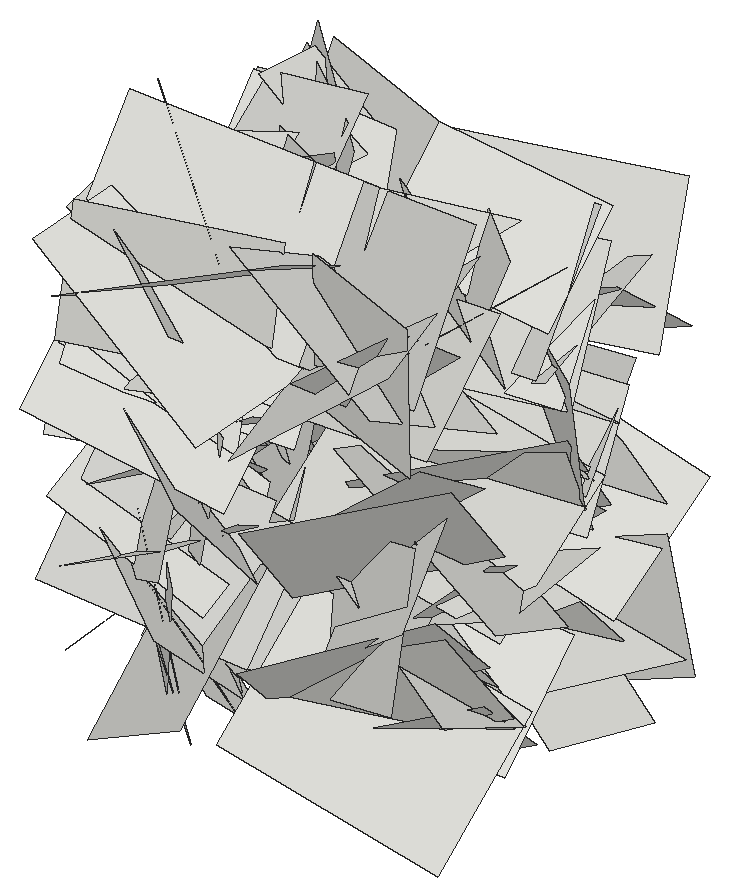
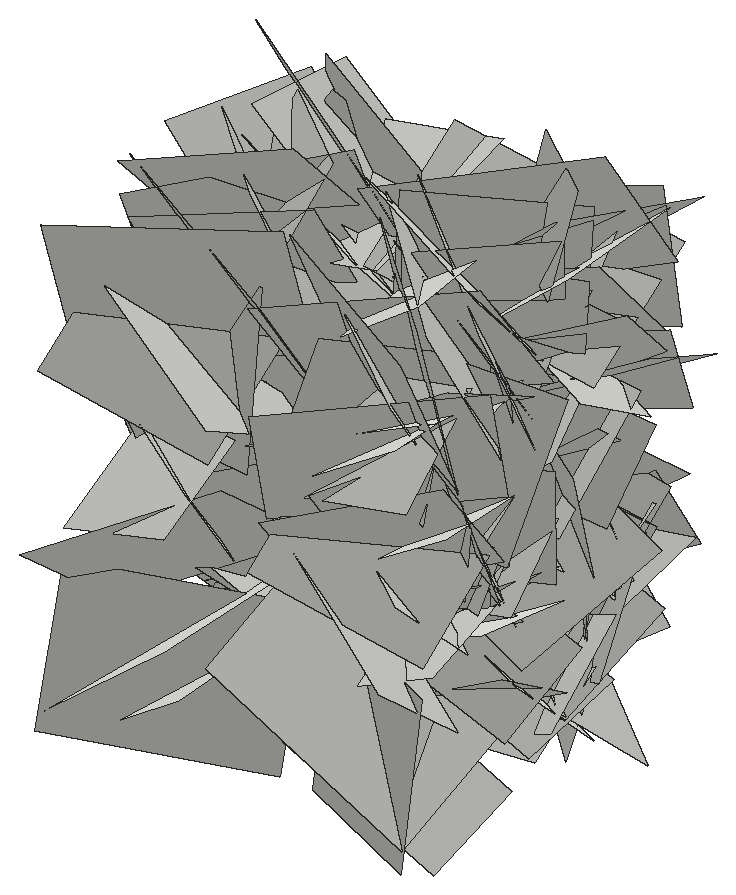
# SketchUp Ruby script. Lengths in inches.
U = 1.inch
M = Sketchup.active_model
def pt(a) = Geom::Point3d.new(a.map { |v| v * U })
def face(e, loops, mat)
  f = e.add_face(loops[0].map { |a| pt(a) })
  loops[1..].each { |l| e.add_face(l.map { |a| pt(a) }).erase! }
  f.material = f.back_material = mat if mat
  f
end
# faces: each face lists its corners as indices into pts; further lists are holes
def faces(e, pts, list, mat = nil) = list.each { |f| face(e, (f[0].is_a?(Array) ? f : [f]).map { |l| l.map { |i| pts[i] } }, mat) }
# xy, xz, yz: faces in a plane at the given z, y or x. An outline is a flat list of corners, or four numbers for a rectangle; further outlines are holes
def ring(l) = l.size == 4 ? [[l[0], l[1]], [l[2], l[1]], [l[2], l[3]], [l[0], l[3]]] : l.each_slice(2).to_a
def flat(e, list, mat, &to3) = list.each { |f| face(e, (f[0].is_a?(Array) ? f : [f]).map { |l| ring(l).map { |u, v| to3.(u, v) } }, mat) }
def xy(e, z, list, mat = nil) = flat(e, list, mat) { |x, y| [x, y, z] }
def xz(e, y, list, mat = nil) = flat(e, list, mat) { |x, z| [x, y, z] }
def yz(e, x, list, mat = nil) = flat(e, list, mat) { |y, z| [x, y, z] }
def lines(e, pts, list) = list.each { |a, b| e.add_line(pt(pts[a]), pt(pts[b])) }
# prism: a flat outline (further loops are holes) pulled along v
def prism(e, loops, v, mat = nil)
  f = face(e, loops, mat); d = Geom::Vector3d.new(v.map { |x| x * U })
  f.pushpull(f.normal.samedirection?(d) ? d.length : -d.length)
end
def box(e, o, s, mat = nil) = prism(e, [[o, [o[0] + s[0], o[1], o[2]], [o[0] + s[0], o[1] + s[1], o[2]], [o[0], o[1] + s[1], o[2]]]], [0, 0, s[2]], mat)
def at(x, y, z, deg = 0) = Geom::Transformation.translation(pt([x, y, z])) * Geom::Transformation.rotation(ORIGIN, Z_AXIS, deg.degrees)
def axes(o, x, y, z) = Geom::Transformation.new([*x, 0, *y, 0, *z, 0, *pt(o).to_a, 1])
def part(name) = M.definitions.add(name)
# library, detail: a bought-in or finely detailed component or shape, given as its bounding box
def library(name, o, s) = part(name).tap { |d| box(d.entities, o, s) }
def detail(e, o, s) = box(e.add_group.entities, o, s)
def put(e, d, t, mat = nil) = e.add_instance(d, t).tap { |i| i.material = mat if mat }
def group(e, t, mat = nil) = e.add_group.tap { |g| g.transformation = t; g.material = mat if mat }.entities
root = M.entities
c1 = part("Component\#6")
p = [[0.01,0,0],[0,3.24,4.54],[4.32,3.24,4.54],[4.33,0,0]]
faces(c1.entities,p,[[0,1,2,3]])
put(root,c1,axes([410.71,164.95,29.96],[-0.04265,0.57286,-0.52342],[0.15347,-0.50938,-0.56862],[0.80809,0.12697,0.08036]))
put(root,c1,axes([410.71,167.51,23.32],[-0.04127,-0.8056,0.43064],[-0.05085,0.43224,0.80425],[0.96695,-0.01165,0.06068]))
put(root,c1,axes([410.71,163.99,40.83],[0.08038,0.23372,-0.81219],[-0.10222,-0.80774,-0.24144],[0.89001,-0.11388,0.04562]))
put(root,c1,axes([410.71,164.8,26.41],[0.06555,-0.88967,-0.10275],[-0.1194,-0.1099,0.88381],[0.94178,0.04799,0.1192]))
put(root,c1,axes([414.68,169.82,24.93],[-0.00586,-0.68753,0.27068],[-0.05817,0.27032,0.6855],[-0.78107,-0.01497,-0.05308]))
put(root,c1,axes([414.68,164.96,33.58],[-0.03363,-0.67551,-0.53197],[0.14584,-0.52946,0.66412],[-0.89967,-0.06058,0.12754]))
put(root,c1,axes([410.71,168.875,35.8],[0.07444,0.7996,-0.0855],[0.00091,-0.0859,-0.80263],[0.85241,-0.06974,0.00832]))
put(root,c1,axes([410.71,164.5,23.79],[0.04443,0.667,0.37408],[0.11412,0.36576,-0.66423],[0.80255,-0.08894,0.07374]))
put(root,c1,axes([410.71,162.92,24.26],[0.16568,0.16434,-0.80239],[-0.1251,-0.80382,-0.18763],[0.85913,-0.14874,0.12742]))
put(root,c1,axes([410.71,162.61,28.57],[-0.04222,-0.49534,0.62953],[0.20196,0.60636,0.48917],[0.82474,-0.17384,-0.08755]))
put(root,c1,axes([410.71,162.43,26.35],[0.02315,-0.70596,0.51236],[-0.01203,0.51225,0.70629],[0.92456,0.02434,-0.00364]))
put(root,c1,axes([414.68,171.89,34.33],[0.10287,-0.74562,-0.1631],[-0.15609,-0.17961,0.73351],[-0.79385,-0.06131,-0.16536]))
put(root,c1,axes([410.71,171.21,38.93],[-0.24063,-0.51313,-1.11059],[-0.16085,-1.10901,0.54342],[1.28679,-0.23458,-0.13976]))
put(root,c1,axes([410.71,166.53,31.68],[-0.02185,0.89564,-0.0065],[0.05171,-0.00537,-0.89456],[0.948,0.02094,0.04865]))
put(root,c1,axes([410.71,158.45,30.92],[-0.16236,0.46297,0.88251],[0.09478,0.89566,-0.45434],[1.05211,-0.00924,0.17712]))
put(root,c1,axes([410.71,163.85,33.45],[-0.03445,-0.73428,-0.4148],[0.17499,-0.41262,0.71747],[0.87664,0.05351,-0.15952]))
put(root,c1,axes([414.68,168.18,25.35],[-0.0356,-0.79141,-0.13903],[0.13499,-0.14264,0.78117],[-0.84098,0.01061,0.13127]))
put(root,c1,axes([414.68,167.69,34.89],[-0.01272,-0.59445,-0.3878],[-0.01652,-0.38754,0.59453],[-0.75216,0.01856,-0.0065]))
put(root,c1,axes([410.71,171.77,39.47],[-0.25632,-0.1505,-1.28885],[-0.2021,-1.29268,0.18672],[1.36053,-0.22038,-0.21508]))
put(root,c1,axes([410.71,166.33,22.3],[-0.05809,-0.87115,0.26873],[0.09257,0.26296,0.87026],[0.96191,-0.07791,-0.06752]))
put(root,c1,axes([410.71,162.32,28.44],[0.12821,-0.42216,-0.69512],[-0.01339,-0.70366,0.42514],[0.86197,0.05186,0.11]))
put(root,c1,axes([414.68,169.92,30.86],[-0.08798,0.07784,-0.70174],[0.08853,-0.70052,-0.08758],[-0.74315,-0.09267,0.07264]))
put(root,c1,axes([410.71,164.2,31.01],[-0.06613,-0.18181,-0.96198],[0.02897,-0.96387,0.1804],[1.03734,0.01533,-0.06637]))
put(root,c1,axes([410.71,161.79,25.53],[0.01152,-0.82607,0.19056],[0.15176,0.18963,0.81386],[0.88572,-0.02175,-0.14193]))
put(root,c1,axes([414.68,169.17,27.35],[-0.00515,-0.4485,-0.48712],[-0.04455,-0.48594,0.44784],[-0.70046,0.0342,-0.02491]))
put(root,c1,axes([414.68,158.39,26.84],[0.02686,0.84806,0.10272],[0.17857,0.09579,-0.83237],[-0.88773,0.04493,-0.16432]))
put(root,c1,axes([410.71,167.34,31.77],[-0.2501,0.51374,1.1242],[-0.05799,1.13903,-0.532],[1.3089,0.14863,0.19123]))
put(root,c1,axes([414.68,159.67,28.14],[0.12868,0.67272,0.52517],[0.08613,0.51893,-0.68352],[-0.90053,0.14576,0.00967]))
put(root,c1,axes([414.68,160.06,22.6],[0.02839,-0.24478,0.77995],[0.15528,0.76918,0.23637],[-0.85248,0.13195,0.06903]))
put(root,c1,axes([414.68,159.46,22.85],[0.09982,-0.0635,0.89488],[0.1784,0.88507,0.04509],[-0.93408,0.16225,0.10424]))
put(root,c1,axes([414.68,168.82,35.84],[-0.04533,0.37689,0.51175],[0.01637,0.51337,-0.3768],[-0.67349,-0.01289,-0.04361]))
put(root,c1,axes([410.71,157.3125,32.29],[-0.25179,1.05256,0.51222],[0.06429,0.53303,-1.06718],[1.23914,0.18623,0.15945]))
put(root,c1,axes([410.71,167.29,35.58],[0.17595,-0.29467,-0.74084],[0.05215,-0.7515,0.30993],[0.84352,0.10793,0.13537]))
put(root,c1,axes([414.68,171.91,32.4],[-0.07209,-0.36069,-0.54144],[0.07785,-0.54516,0.35394],[-0.6852,-0.024,0.09718]))
put(root,c1,axes([410.71,165.04,27.71],[-0.04822,0.07219,0.94774],[0.14201,0.93984,-0.06516],[0.99746,-0.13032,0.05509]))
put(root,c1,axes([414.68,162.33,29.83],[0.22776,0.38392,-0.75072],[-0.01782,-0.77261,-0.39993],[-0.89361,0.11326,-0.18337]))
put(root,c1,axes([414.68,168.23,31.98],[0.11552,-0.73847,0.10601],[-0.00435,0.10653,0.74638],[-0.79079,-0.10846,0.01138]))
put(root,c1,axes([410.71,159.15,32.85],[-0.28722,0.93511,0.86971],[-0.00467,0.88838,-0.95656],[1.35365,0.20148,0.18123]))
put(root,c1,axes([414.68,170.38,37.22],[0.01844,-0.65259,0.06973],[0.0154,0.07012,0.65262],[-0.69551,-0.01575,0.0163]))
put(root,c1,axes([410.71,162.15,25.43],[-0.09766,0.84172,-0.54191],[0.18116,-0.52299,-0.84139],[1.04557,0.16923,0.09516]))
put(root,c1,axes([414.68,165.16,26.22],[-0.00662,-0.41647,0.48084],[0.04981,0.47925,0.41571],[-0.67246,0.0396,0.02606]))
put(root,c1,axes([414.68,166.74,28.03],[0.20581,0.5378,0.53941],[-0.0447,0.5634,-0.54654],[-0.80617,0.10606,0.16802]))
put(root,c1,axes([414.68,167.3,30.05],[0.09755,-0.36279,0.79394],[0.2327,0.7823,0.33203],[-0.89554,0.16375,0.17276]))
put(root,c1,axes([414.68,163.79,31.02],[0.0186,-0.39942,0.51021],[0.04828,0.50989,0.39761],[-0.68514,0.02509,0.04187]))
put(root,c1,axes([414.68,168.24,29.62],[0.00844,-0.1319,-0.59476],[0.00779,-0.59475,0.132],[-0.64572,-0.0089,-0.00618]))
put(root,c1,axes([410.71,168.37,37.02],[-0.06582,-0.55881,-0.84289],[0.17414,-0.83883,0.54402],[1.05774,0.10333,-0.14201]))
put(root,c1,axes([410.71,162.55,24.47],[0.08094,0.6993,-0.63815],[0.06519,-0.64254,-0.69674],[1.00139,-0.01469,0.09694]))
put(root,c1,axes([414.68,167.47,38.84],[0.19203,-0.25676,-0.78485],[0.09527,-0.79261,0.28005],[-0.87013,-0.14344,-0.14255]))
put(root,c1,axes([414.68,168.14,25.37],[0.00005,-0.54267,0.44601],[0.16088,0.43548,0.52984],[-0.72699,0.09633,0.11728]))
put(root,c1,axes([410.71,169.13,31.47],[0.22896,-0.22184,-0.76377],[0.12794,-0.77313,0.25869],[0.83329,0.17965,0.17014]))
put(root,c1,axes([410.71,164.67,22.86],[-0.07455,-1.03669,0.46758],[0.01691,0.46753,1.03897],[1.20537,-0.07068,0.01434]))
put(root,c1,axes([414.68,161.42,33.85],[0.12931,-0.58697,0.4315],[0.06321,0.44408,0.58723],[-0.76963,-0.06214,0.12073]))
put(root,c1,axes([410.71,160.7,27.63],[-0.09928,0.64406,-0.88513],[0.13228,-0.87629,-0.65083],[1.15276,0.15602,-0.00154]))
put(root,c1,axes([410.71,159.57,38.3125],[-0.19748,1.37219,0.09956],[-0.15298,0.08042,-1.37849],[1.4503,0.19533,-0.13185]))
put(root,c1,axes([414.68,165.91,24.52],[-0.03596,-0.58924,0.24858],[0.15481,0.23521,0.57749],[-0.65999,0.08727,0.12191]))
put(root,c1,axes([410.71,166.55,31.56],[0.0814,0.41102,-0.8284],[0.17089,-0.82447,-0.39413],[0.96524,0.11131,0.13964]))
put(root,c1,axes([414.68,169.1,21.1],[0.05323,-0.42134,0.48328],[0.06346,0.48572,0.41725],[-0.67666,0.01241,0.07715]))
put(root,c1,axes([410.71,166.67,25.47],[-0.29316,-1.18227,0.54308],[0.10516,0.53443,1.21398],[1.37509,-0.29293,0.02294]))
put(root,c1,axes([410.71,168.75,37.98],[-0.06882,-0.53698,-1.12739],[-0.1022,-1.12338,0.54063],[1.31971,-0.115,-0.01692]))
put(root,c1,axes([410.71,158.58,28.72],[0.17742,0.80309,0.64454],[-0.10421,0.66248,-0.79991],[1.08655,-0.0676,-0.18196]))
put(root,c1,axes([414.68,163.1,21.29],[0.03251,-0.459,0.52355],[0.17075,0.51451,0.44164],[-0.71801,0.10157,0.12873]))
put(root,c1,axes([410.71,169.04,36.23],[-0.04162,0.78981,-0.64322],[0.24351,-0.62024,-0.77563],[1.05189,0.17484,0.15411]))
put(root,c1,axes([410.71,170.89,20.28],[0.12274,-1.02279,0.17958],[-0.0333,0.17716,1.02926],[1.10024,0.11946,0.01112]))
put(root,c1,axes([410.71,167.53,29.6],[0.04916,0.6172,0.8297],[0.08211,0.82613,-0.61887],[1.09305,-0.08981,0.00917]))
put(root,c1,axes([410.71,171.44,27.64],[0.05126,-0.8571,0.56567],[0.11133,0.56746,0.85083],[1.08285,-0.01777,-0.11425]))
put(root,c1,axes([414.68,163.13,28.77],[0.13219,-0.55975,0.33448],[0.05965,0.34851,0.56225],[-0.68862,-0.07726,0.11291]))
put(root,c1,axes([410.71,163.625,35.04],[0.27654,-0.44632,0.88094],[-0.09901,0.89592,0.48157],[1.04211,0.20356,-0.18801]))
put(root,c1,axes([410.71,167.41,29.34],[-0.20833,-0.42173,1.22713],[0.0869,1.23461,0.43743],[1.37269,-0.14217,0.15855]))
put(root,c1,axes([410.71,168.84,39.14],[0.0295,-0.69575,-0.73723],[0.22295,-0.71749,0.68506],[1.05113,0.17171,-0.12461]))
put(root,c1,axes([410.71,163.85,26.9],[0.03329,1.04875,0.11229],[0.24045,0.10299,-1.02538],[1.09187,-0.05466,0.22238]))
put(root,c1,axes([410.71,160.22,28.4],[0.15479,0.80897,-0.76348],[-0.02106,-0.76802,-0.81757],[1.17891,-0.11994,0.08565]))
put(root,c1,axes([410.71,169.63,32.59],[0.01533,-0.4611,-1.03377],[0.17767,-1.02158,0.45801],[1.18663,0.15892,-0.05522]))
put(root,c1,axes([410.71,159.8,34.2],[-0.03301,0.77795,0.85676],[0.24326,0.8442,-0.75821],[1.20233,-0.14944,0.17692]))
put(root,c1,axes([410.71,166.97,25.06],[-0.03339,-0.82276,-0.77538],[0.30966,-0.75526,0.78954],[1.15769,0.17829,-0.23355]))
put(root,c1,axes([410.71,165.55,34.43],[-0.04885,1.13911,0.54464],[0.08516,0.54654,-1.13629],[1.33566,0.00681,0.09237]))
put(root,c1,axes([410.71,164.92,23.28],[0.02573,-1.02703,-0.88101],[-0.12942,-0.87922,1.02158],[1.42847,-0.06116,0.10843]))
put(root,c1,axes([410.71,160.96,32.62],[0.12215,0.75895,-0.88724],[0.014,-0.89234,-0.7616],[1.23753,-0.06482,0.09619]))
put(root,c1,axes([410.71,172.54,38.57],[-0.12011,-0.4932,-1.18141],[0.20578,-1.17893,0.47355],[1.34134,0.1367,-0.17844]))
put(root,c1,axes([410.71,171.44,26.6],[-0.03428,0.27698,-1.26013],[0.06702,-1.25867,-0.27828],[1.36598,0.0687,-0.01797]))
put(root,c1,axes([410.71,173.53,27.66],[0.08068,-0.97468,-0.75893],[0.01331,-0.75972,0.97695],[1.30935,0.06778,0.03684]))
put(root,c1,axes([410.71,158.99,33.95],[0.09747,0.08794,1.12692],[0.17247,1.11783,-0.1005],[1.18568,-0.16983,-0.07802]))
put(root,c1,axes([410.71,166.62,31.96],[0.21061,0.75098,-0.921],[-0.02022,-0.93165,-0.76377],[1.25951,-0.14053,0.14175]))
put(root,c1,axes([410.71,158.06,26.05],[0.19995,0.52409,1.06255],[0.00833,1.07535,-0.5318],[1.25583,-0.09057,-0.16565]))
put(root,c1,axes([410.71,172.42,21.79],[0.22827,-1.35966,0.24048],[-0.1567,0.21929,1.3722],[1.45519,0.2369,0.11004]))
put(root,c1,axes([410.71,165.11,34.6875],[0.03998,0.77126,1.05992],[0.2457,1.03973,-0.76482],[1.36759,-0.20934,0.10642]))
put(root,c1,axes([410.71,159.18,36.25],[0.04304,0.74935,1.15311],[0.14712,1.14549,-0.74928],[1.45028,-0.13844,0.04179]))
put(root,c1,axes([410.71,168.45,29.92],[0.2904,-0.81126,-1.09363],[-0.15157,-1.12651,0.79984],[1.4354,0.04517,0.30571]))
put(root,c1,axes([410.71,157.9,37.93],[0.24747,1.3445,0.30187],[-0.11522,0.32319,-1.35538],[1.4561,-0.20293,-0.15855]))
put(root,c1,axes([410.71,163.2,33.68],[0.16473,-1.2102,0.57798],[0.2383,0.59712,1.18983],[1.40149,0.04071,-0.27024]))
put(root,c1,axes([424.49,163.2,33.68],[-0.16473,-1.2102,0.57798],[-0.2383,0.59712,1.18983],[-1.40149,0.04071,-0.27024]))
put(root,c1,axes([424.49,157.9,37.93],[-0.24747,1.3445,0.30187],[0.11522,0.32319,-1.35538],[-1.4561,-0.20293,-0.15855]))
put(root,c1,axes([424.49,168.45,29.92],[-0.2904,-0.81126,-1.09363],[0.15157,-1.12651,0.79984],[-1.4354,0.04517,0.30571]))
put(root,c1,axes([424.49,159.18,36.25],[-0.04304,0.74935,1.15311],[-0.14712,1.14549,-0.74928],[-1.45028,-0.13844,0.04179]))
put(root,c1,axes([424.49,165.11,34.6875],[-0.03998,0.77126,1.05992],[-0.2457,1.03973,-0.76482],[-1.36759,-0.20934,0.10642]))
put(root,c1,axes([424.49,172.42,21.79],[-0.22827,-1.35966,0.24048],[0.1567,0.21929,1.3722],[-1.45519,0.2369,0.11004]))
put(root,c1,axes([424.49,158.06,26.05],[-0.19995,0.52409,1.06255],[-0.00833,1.07535,-0.5318],[-1.25583,-0.09057,-0.16565]))
put(root,c1,axes([424.49,166.62,31.96],[-0.21061,0.75098,-0.921],[0.02022,-0.93165,-0.76377],[-1.25951,-0.14053,0.14175]))
put(root,c1,axes([424.49,158.99,33.95],[-0.09747,0.08794,1.12692],[-0.17247,1.11783,-0.1005],[-1.18568,-0.16983,-0.07802]))
put(root,c1,axes([424.49,173.53,27.66],[-0.08068,-0.97468,-0.75893],[-0.01331,-0.75972,0.97695],[-1.30935,0.06778,0.03684]))
put(root,c1,axes([424.49,171.44,26.6],[0.03428,0.27698,-1.26013],[-0.06702,-1.25867,-0.27828],[-1.36598,0.0687,-0.01797]))
put(root,c1,axes([424.49,172.54,38.57],[0.12011,-0.4932,-1.18141],[-0.20578,-1.17893,0.47355],[-1.34134,0.1367,-0.17844]))
put(root,c1,axes([424.49,160.96,32.62],[-0.12215,0.75895,-0.88724],[-0.014,-0.89234,-0.7616],[-1.23753,-0.06482,0.09619]))
put(root,c1,axes([424.49,164.92,23.28],[-0.02573,-1.02703,-0.88101],[0.12942,-0.87922,1.02158],[-1.42847,-0.06116,0.10843]))
put(root,c1,axes([424.49,165.55,34.43],[0.04885,1.13911,0.54464],[-0.08516,0.54654,-1.13629],[-1.33566,0.00681,0.09237]))
put(root,c1,axes([424.49,166.97,25.06],[0.03339,-0.82276,-0.77538],[-0.30966,-0.75526,0.78954],[-1.15769,0.17829,-0.23355]))
put(root,c1,axes([424.49,159.8,34.2],[0.03301,0.77795,0.85676],[-0.24326,0.8442,-0.75821],[-1.20233,-0.14944,0.17692]))
put(root,c1,axes([424.49,169.63,32.59],[-0.01533,-0.4611,-1.03377],[-0.17767,-1.02158,0.45801],[-1.18663,0.15892,-0.05522]))
put(root,c1,axes([424.49,160.22,28.4],[-0.15479,0.80897,-0.76348],[0.02106,-0.76802,-0.81757],[-1.17891,-0.11994,0.08565]))
put(root,c1,axes([424.49,163.85,26.9],[-0.03329,1.04875,0.11229],[-0.24045,0.10299,-1.02538],[-1.09187,-0.05466,0.22238]))
put(root,c1,axes([424.49,168.84,39.14],[-0.0295,-0.69575,-0.73723],[-0.22295,-0.71749,0.68506],[-1.05113,0.17171,-0.12461]))
put(root,c1,axes([424.49,167.41,29.34],[0.20833,-0.42173,1.22713],[-0.0869,1.23461,0.43743],[-1.37269,-0.14217,0.15855]))
put(root,c1,axes([424.49,163.625,35.04],[-0.27654,-0.44632,0.88094],[0.09901,0.89592,0.48157],[-1.04211,0.20356,-0.18801]))
put(root,c1,axes([420.52,163.13,28.77],[-0.13219,-0.55975,0.33448],[-0.05965,0.34851,0.56225],[0.68862,-0.07726,0.11291]))
put(root,c1,axes([424.49,171.44,27.64],[-0.05126,-0.8571,0.56567],[-0.11133,0.56746,0.85083],[-1.08285,-0.01777,-0.11425]))
put(root,c1,axes([424.49,167.53,29.6],[-0.04916,0.6172,0.8297],[-0.08211,0.82613,-0.61887],[-1.09305,-0.08981,0.00917]))
put(root,c1,axes([424.49,170.89,20.28],[-0.12274,-1.02279,0.17958],[0.0333,0.17716,1.02926],[-1.10024,0.11946,0.01112]))
put(root,c1,axes([424.49,169.04,36.23],[0.04162,0.78981,-0.64322],[-0.24351,-0.62024,-0.77563],[-1.05189,0.17484,0.15411]))
put(root,c1,axes([420.52,163.1,21.29],[-0.03251,-0.459,0.52355],[-0.17075,0.51451,0.44164],[0.71801,0.10157,0.12873]))
put(root,c1,axes([424.49,158.58,28.72],[-0.17742,0.80309,0.64454],[0.10421,0.66248,-0.79991],[-1.08655,-0.0676,-0.18196]))
put(root,c1,axes([424.49,168.75,37.98],[0.06882,-0.53698,-1.12739],[0.1022,-1.12338,0.54063],[-1.31971,-0.115,-0.01692]))
put(root,c1,axes([424.49,166.67,25.47],[0.29316,-1.18227,0.54308],[-0.10516,0.53443,1.21398],[-1.37509,-0.29293,0.02294]))
put(root,c1,axes([420.52,169.1,21.1],[-0.05323,-0.42134,0.48328],[-0.06346,0.48572,0.41725],[0.67666,0.01241,0.07715]))
put(root,c1,axes([424.49,166.55,31.56],[-0.0814,0.41102,-0.8284],[-0.17089,-0.82447,-0.39413],[-0.96524,0.11131,0.13964]))
put(root,c1,axes([420.52,165.91,24.52],[0.03596,-0.58924,0.24858],[-0.15481,0.23521,0.57749],[0.65999,0.08727,0.12191]))
put(root,c1,axes([424.49,159.57,38.3125],[0.19748,1.37219,0.09956],[0.15298,0.08042,-1.37849],[-1.4503,0.19533,-0.13185]))
put(root,c1,axes([424.49,160.7,27.63],[0.09928,0.64406,-0.88513],[-0.13228,-0.87629,-0.65083],[-1.15276,0.15602,-0.00154]))
put(root,c1,axes([420.52,161.42,33.85],[-0.12931,-0.58697,0.4315],[-0.06321,0.44408,0.58723],[0.76963,-0.06214,0.12073]))
put(root,c1,axes([424.49,164.67,22.86],[0.07455,-1.03669,0.46758],[-0.01691,0.46753,1.03897],[-1.20537,-0.07068,0.01434]))
put(root,c1,axes([424.49,169.13,31.47],[-0.22896,-0.22184,-0.76377],[-0.12794,-0.77313,0.25869],[-0.83329,0.17965,0.17014]))
put(root,c1,axes([420.52,168.14,25.37],[-0.00005,-0.54267,0.44601],[-0.16088,0.43548,0.52984],[0.72699,0.09633,0.11728]))
put(root,c1,axes([420.52,167.47,38.84],[-0.19203,-0.25676,-0.78485],[-0.09527,-0.79261,0.28005],[0.87013,-0.14344,-0.14255]))
put(root,c1,axes([424.49,162.55,24.47],[-0.08094,0.6993,-0.63815],[-0.06519,-0.64254,-0.69674],[-1.00139,-0.01469,0.09694]))
put(root,c1,axes([424.49,168.37,37.02],[0.06582,-0.55881,-0.84289],[-0.17414,-0.83883,0.54402],[-1.05774,0.10333,-0.14201]))
